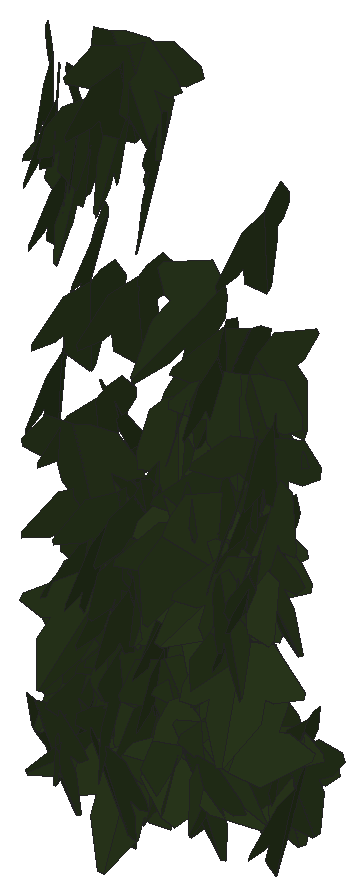
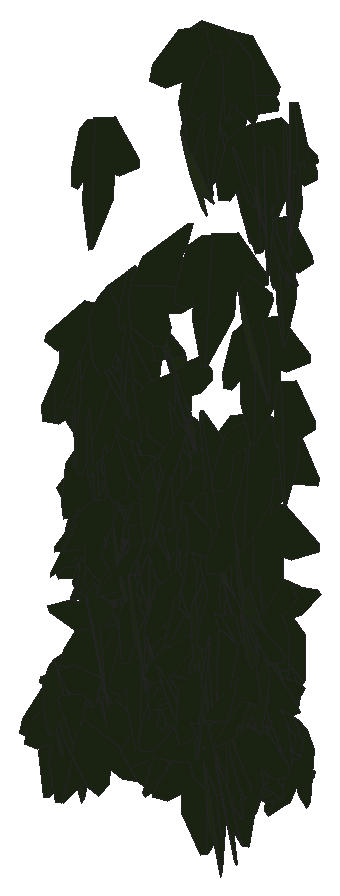
# SketchUp Ruby script. Lengths in inches.
U = 1.inch
M = Sketchup.active_model
def pt(a) = Geom::Point3d.new(a.map { |v| v * U })
def face(e, loops, mat)
  f = e.add_face(loops[0].map { |a| pt(a) })
  loops[1..].each { |l| e.add_face(l.map { |a| pt(a) }).erase! }
  f.material = f.back_material = mat if mat
  f
end
# faces: each face lists its corners as indices into pts; further lists are holes
def faces(e, pts, list, mat = nil) = list.each { |f| face(e, (f[0].is_a?(Array) ? f : [f]).map { |l| l.map { |i| pts[i] } }, mat) }
# xy, xz, yz: faces in a plane at the given z, y or x. An outline is a flat list of corners, or four numbers for a rectangle; further outlines are holes
def ring(l) = l.size == 4 ? [[l[0], l[1]], [l[2], l[1]], [l[2], l[3]], [l[0], l[3]]] : l.each_slice(2).to_a
def flat(e, list, mat, &to3) = list.each { |f| face(e, (f[0].is_a?(Array) ? f : [f]).map { |l| ring(l).map { |u, v| to3.(u, v) } }, mat) }
def xy(e, z, list, mat = nil) = flat(e, list, mat) { |x, y| [x, y, z] }
def xz(e, y, list, mat = nil) = flat(e, list, mat) { |x, z| [x, y, z] }
def yz(e, x, list, mat = nil) = flat(e, list, mat) { |y, z| [x, y, z] }
def lines(e, pts, list) = list.each { |a, b| e.add_line(pt(pts[a]), pt(pts[b])) }
# prism: a flat outline (further loops are holes) pulled along v
def prism(e, loops, v, mat = nil)
  f = face(e, loops, mat); d = Geom::Vector3d.new(v.map { |x| x * U })
  f.pushpull(f.normal.samedirection?(d) ? d.length : -d.length)
end
def box(e, o, s, mat = nil) = prism(e, [[o, [o[0] + s[0], o[1], o[2]], [o[0] + s[0], o[1] + s[1], o[2]], [o[0], o[1] + s[1], o[2]]]], [0, 0, s[2]], mat)
def at(x, y, z, deg = 0) = Geom::Transformation.translation(pt([x, y, z])) * Geom::Transformation.rotation(ORIGIN, Z_AXIS, deg.degrees)
def axes(o, x, y, z) = Geom::Transformation.new([*x, 0, *y, 0, *z, 0, *pt(o).to_a, 1])
def part(name) = M.definitions.add(name)
# library, detail: a bought-in or finely detailed component or shape, given as its bounding box
def library(name, o, s) = part(name).tap { |d| box(d.entities, o, s) }
def detail(e, o, s) = box(e.add_group.entities, o, s)
def put(e, d, t, mat = nil) = e.add_instance(d, t).tap { |i| i.material = mat if mat }
def group(e, t, mat = nil) = e.add_group.tap { |g| g.transformation = t; g.material = mat if mat }.entities
root = M.entities
M.materials.add("efeu2").color = [43, 57, 29]
c1 = part("ivyleaf_10")
p = [[0,0.5,-0.03],[-0.0625,2.02,-0.43],[-0.19,2.01,-0.46],[-0.54,1.05,-0.29],[-0.52,0.625,-0.18],[-0.83,0.76,-0.28],
  [-1.16,0.64,-0.33],[-1.15,0.33,-0.24],[-0.77,-0.39,0.02],[-0.3,-0.51,0.16],[0.04,-0.48,0.23],[-0.02,2.01,-0.4375],
  [-0.06,2.01,-0.43],[0.04,-0.49,0.23],[0.67,-0.49,0.14],[1.38,0.36,-0.2],[1.375,0.51,-0.24],[0.81,0.65,-0.19],
  [0.62,0.59,-0.15],[0.6,1.09,-0.28],[0.5,1.23,-0.31]]
faces(c1.entities,p,[[0,1,2,3,4,5,6,7,8,9,10],[11,12,0,13,14,15,16,17,18,19,20]],"efeu2")
put(root,c1,axes([515.31,136.94,182.59],[0.33871,-0.54812,-0.3443],[-0.05591,0.36236,-0.63188],[0.64487,0.31931,0.12606]))
put(root,c1,axes([515.36,137.18,180.82],[0.18828,-0.62964,-0.25162],[-0.048,0.24811,-0.65677],[0.67636,0.19288,0.02343]))
put(root,c1,axes([515.2,137.09,172.68],[-0.54988,0.28475,-0.17468],[0.14668,-0.09646,-0.61899],[-0.30013,-0.56884,0.01753]))
put(root,c1,axes([515.38,137.06,178.12],[0.1741,-0.59957,-0.27894],[-0.04764,0.27633,-0.62369],[0.65957,0.17823,0.02858]))
put(root,c1,axes([515.23,137.99,174.27],[-0.51868,0.3402,-0.19325],[0.15254,-0.11968,-0.6201],[-0.3603,-0.54042,0.01567]))
put(root,c1,axes([515.52,137.77,173.53],[0.349,0.37677,-0.38742],[-0.30336,-0.24507,-0.51163],[-0.44724,0.46025,0.04472]))
put(root,c1,axes([515.37,137.59,173.74],[0.19264,0.60685,0.10715],[-0.1052,0.143,-0.62076],[-0.6072,0.16775,0.14154]))
put(root,c1,axes([515.47,137.55,173.92],[0.58092,-0.27653,-0.19393],[-0.16516,0.10397,-0.643],[0.29462,0.60354,0.02192]))
put(root,c1,axes([515.51,136.77,182.11],[0.22554,-0.59634,-0.35365],[-0.08086,0.34673,-0.63624],[0.68859,0.23604,0.04113]))
put(root,c1,axes([515.46,137.56,175.03],[0.13649,-0.64431,0.12548],[0.01418,-0.12524,-0.6585],[0.65626,0.13671,-0.01187]))
put(root,c1,axes([515.33,137.76,173.71],[-0.01707,0.63833,-0.12351],[0.01068,-0.12326,-0.63852],[-0.65008,-0.01879,-0.00725]))
put(root,c1,axes([515.5625,137.21,181.9],[0.35337,-0.44125,-0.43697],[-0.13703,0.43497,-0.55004],[0.60569,0.35584,0.13049]))
put(root,c1,axes([515.51,137.68,173.05],[0.08292,-0.59778,0.32093],[0.07529,-0.31322,-0.60286],[0.6743,0.10849,0.02785]))
put(root,c1,axes([515.46,138.07,173.1],[0.64257,0.11943,0.00816],[-0.00384,0.0651,-0.65037],[-0.11964,0.63932,0.0647]))
put(root,c1,axes([515.57,137.65,179.83],[0.32215,-0.60836,0.03694],[0.03103,-0.02536,-0.68821],[0.60869,0.32327,0.01554]))
put(root,c1,axes([515.53,138.28,172.5],[0.42789,-0.48623,0.05749],[0.08214,-0.00397,-0.64502],[0.48268,0.43172,0.05881]))
put(root,c1,axes([515.49,137.3125,181.13],[0.55305,-0.41382,0.16129],[0.12199,-0.10614,-0.69064],[0.42706,0.56623,-0.01158]))
put(root,c1,axes([515.68,137.93,174.3],[-0.62471,0.18782,0.04065],[-0.03909,0.0112,-0.65233],[-0.18815,-0.62593,0.00053]))
put(root,c1,axes([515.69,137.32,179.13],[-0.09387,-0.66963,-0.14527],[0.02357,0.14338,-0.67617],[0.6848,-0.09673,0.00336]))
put(root,c1,axes([515.74,137.77,174.64],[0.59877,-0.12566,-0.22355],[-0.22194,0.03057,-0.61164],[0.12849,0.63841,-0.01471]))
put(root,c1,axes([515.85,137.69,173.08],[-0.57795,-0.24468,0.20168],[-0.16829,-0.11866,-0.62624],[0.26874,-0.60052,0.04156]))
put(root,c1,axes([515.96,137.73,172.47],[0.05075,0.24534,-0.60965],[-0.49643,-0.38635,-0.1968],[-0.43061,0.47432,0.15504]))
put(root,c1,axes([515.74,137.32,176.09],[-0.32489,-0.60884,-0.06624],[0.02845,0.05989,-0.69009],[0.61177,-0.32612,-0.00308]))
put(root,c1,axes([515.84,137.22,174.62],[-0.28005,-0.48958,0.37395],[-0.084,-0.37659,-0.55595],[0.6103,-0.27649,0.09508]))
put(root,c1,axes([515.79,137.34,177.41],[-0.13119,-0.65979,-0.19016],[0.02665,0.18856,-0.67263],[0.68613,-0.13348,-0.01023]))
put(root,c1,axes([515.76,137.78,175.13],[0.48977,-0.45924,-0.02017],[-0.00862,0.02029,-0.67134],[0.4596,0.48977,0.0089]))
put(root,c1,axes([515.79,138.23,172.36],[0.2756,-0.58774,-0.07754],[0.01238,0.0912,-0.64726],[0.59271,0.27138,0.04957]))
put(root,c1,axes([515.77,138.22,173.11],[0.54445,0.33969,-0.08162],[-0.08031,-0.02539,-0.64139],[-0.34,0.54995,0.0208]))
put(root,c1,axes([515.92,137.05,182.08],[-0.16433,-0.70047,-0.06187],[0.01857,0.05919,-0.71947],[0.70295,-0.16531,0.00455]))
put(root,c1,axes([515.96,136.84,177.25],[-0.68545,-0.12976,-0.01894],[0.0189,0.00199,-0.69762],[0.12976,-0.68571,0.00156]))
put(root,c1,axes([515.99,138.04,173.74],[-0.14545,-0.63951,0.10688],[0.0004,-0.10962,-0.65539],[0.64838,-0.14339,0.02438]))
put(root,c1,axes([516.13,138.01,174.14],[-0.40383,0.39671,0.35406],[-0.29855,0.19874,-0.5632],[-0.44001,-0.49894,0.05718]))
put(root,c1,axes([516.05,138.08,172.52],[-0.57007,-0.29009,0.06256],[-0.04937,-0.0409,-0.63948],[0.29262,-0.57204,0.01399]))
put(root,c1,axes([516.02,137.14,175.65],[0.23214,-0.67517,-0.16839],[-0.0297,0.16773,-0.7135],[0.69522,0.23261,0.02574]))
put(root,c1,axes([516.09,137.77,173.36],[-0.63952,-0.08182,0.08241],[-0.07285,-0.07655,-0.64133],[0.09043,-0.64025,0.06615]))
put(root,c1,axes([516.07,137.54,174.79],[-0.01294,-0.62664,-0.24537],[0.03214,0.24456,-0.62627],[0.6722,-0.02376,0.02522]))
put(root,c1,axes([516.14,138.02,174.81],[0.2194,-0.62079,-0.10657],[0.00444,0.11437,-0.6571],[0.62986,0.21544,0.04176]))
put(root,c1,axes([516.25,137.29,176.19],[-0.34841,-0.57057,-0.12086],[0.05321,0.1091,-0.66844],[0.5808,-0.35227,-0.01126]))
put(root,c1,axes([516.38,137.875,173.91],[-0.38278,-0.5273,0.0378],[-0.02134,-0.03121,-0.65159],[0.52822,-0.38337,0.00106]))
put(root,c1,axes([516.26,137.2,182],[0.52787,-0.47279,-0.01699],[0.0045,0.03047,-0.70818],[0.47307,0.52726,0.02569]))
put(root,c1,axes([516.09,137.51,173.46],[0.23481,-0.45598,0.45044],[0.28413,-0.35595,-0.50845],[0.57453,0.36239,0.06735]))
put(root,c1,axes([515.97,137.84,176.6875],[-0.42605,0.12559,0.55668],[0.5071,-0.23535,0.44119],[0.26177,0.66032,0.05137]))
put(root,c1,axes([516.33,136.99,172.51],[-0.57322,0.29702,-0.00692],[0.00683,-0.00187,-0.6456],[-0.29702,-0.57326,-0.00148]))
put(root,c1,axes([516.75,137.3125,176.05],[-0.44733,0.03746,-0.51049],[-0.50777,0.05308,0.44884],[0.06459,0.67667,-0.00695]))
put(root,c1,axes([516.29,137.35,172.19],[0.71633,-0.04816,-0.04057],[-0.03949,0.01731,-0.7178],[0.04905,0.71727,0.0146]))
put(root,c1,axes([516.44,138.03,173.33],[-0.3324,-0.57437,0.05078],[0.02629,-0.07365,-0.66095],[0.57602,-0.32809,0.05947]))
put(root,c1,axes([516.31,137.68,172.94],[0.07524,0.3696,0.54415],[0.01485,0.54661,-0.37332],[-0.65764,0.05463,0.05383]))
put(root,c1,axes([516.47,137.21,174.89],[0.05804,-0.57536,-0.35999],[0.03521,0.36337,-0.57509],[0.67779,0.03039,0.0607]))
put(root,c1,axes([516.43,137.33,175.47],[-0.20436,-0.50261,-0.45725],[0.16344,0.4271,-0.54251],[0.65953,-0.26157,-0.00724]))
put(root,c1,axes([517,137.38,174.7],[0.09853,0.07319,-0.70142],[-0.70214,0.0764,-0.09066],[0.06593,0.70418,0.08274]))
put(root,c1,axes([516.51,137.99,175.35],[0.09012,0.55236,-0.35938],[-0.12441,-0.34194,-0.55675],[-0.64713,0.14266,0.05699]))
put(root,c1,axes([516.6,136.85,182.93],[-0.10855,-0.66403,-0.28612],[0.0283,0.2852,-0.67263],[0.72249,-0.11094,-0.01664]))
put(root,c1,axes([516.43,137.83,173.96],[-0.21607,-0.49266,-0.36988],[0.24805,0.28922,-0.53013],[0.56391,-0.31599,0.09146]))
put(root,c1,axes([516.6,137.25,176.36],[-0.12219,-0.5641,-0.39116],[0.09299,0.38004,-0.57712],[0.68012,-0.15331,0.00863]))
put(root,c1,axes([516.63,137.64,173.25],[-0.06443,-0.59383,-0.28635],[0.07386,0.2794,-0.59604],[0.65512,-0.0899,0.03904]))
put(root,c1,axes([516.59,138.08,173.53],[0.6626,-0.01612,-0.00916],[-0.0091,0.00268,-0.66279],[0.01616,0.66265,0.00246]))
put(root,c1,axes([516.875,137.71,177.12],[-0.27266,0.39824,0.45446],[-0.26,0.37274,-0.48263],[-0.54546,-0.37675,0.00288]))
put(root,c1,axes([516.64,136.91,183.27],[-0.674,0.13808,-0.21923],[0.19219,-0.1433,-0.68112],[-0.17375,-0.69412,0.097]))
put(root,c1,axes([516.87,137.97,176.09],[0.61823,0.04994,-0.24838],[-0.25131,0.20381,-0.58455],[0.03208,0.63432,0.20737]))
put(root,c1,axes([516.83,136.875,183.25],[-0.60221,-0.37852,-0.095],[0.0687,0.06915,-0.71095],[0.38416,-0.60572,-0.02179]))
put(root,c1,axes([516.89,136.82,179.84],[-0.11494,-0.69555,-0.19295],[0.03206,0.19027,-0.70498],[0.72111,-0.11932,0.00059]))
put(root,c1,axes([516.71,138.24,173.8125],[0.50861,-0.37359,0.17246],[0.1402,-0.10045,-0.63107],[0.38686,0.52758,0.00197]))
put(root,c1,axes([517.09,137.91,172.15],[0.11225,0.27553,0.57456],[-0.23243,-0.52551,0.29741],[0.59331,-0.258,0.00781]))
put(root,c1,axes([516.98,137.92,176.64],[0.07944,-0.65598,0.04507],[0.00925,-0.04428,-0.66076],[0.65746,0.07988,0.00385]))
put(root,c1,axes([517.03,137.17,174.21],[0.19579,-0.55272,-0.3456],[-0.03576,0.3512,-0.58194],[0.65089,0.18556,0.07198]))
put(root,c1,axes([517.0625,137.38,174.79],[0.13093,-0.64723,-0.20686],[-0.04903,0.20112,-0.66029],[0.67771,0.13959,-0.00781]))
put(root,c1,axes([517,137.93,175.19],[-0.5254,-0.35416,-0.188],[0.14126,0.12652,-0.63313],[0.37526,-0.54349,-0.02488]))
put(root,c1,axes([517.12,137.18,172.875],[0.44878,-0.44902,-0.14413],[-0.09723,0.10658,-0.63481],[0.46146,0.45915,0.00641]))
put(root,c1,axes([517.15,137.9,176.62],[-0.60853,0.26913,0.0819],[-0.06744,0.04992,-0.66513],[-0.27311,-0.61198,-0.01824]))
put(root,c1,axes([516.9,137.28,181.91],[0.35879,-0.49456,0.39986],[0.2629,-0.3027,-0.61029],[0.5791,0.44384,0.02932]))
put(root,c1,axes([517.18,137.47,175.08],[-0.02902,-0.59884,-0.35837],[0.03346,0.35707,-0.59938],[0.69708,-0.04207,0.01385]))
put(root,c1,axes([517.23,137.96,173.86],[-0.10834,-0.62211,-0.16859],[0.01456,0.16855,-0.63131],[0.64438,-0.10841,-0.01408]))
put(root,c1,axes([517.29,137.3,176.04],[-0.26212,-0.59598,0.10222],[0.01025,-0.11577,-0.64872],[0.6046,-0.25642,0.05531]))
put(root,c1,axes([517.3125,138.02,174.8125],[0.26285,-0.58889,-0.16814],[-0.04203,0.1652,-0.64428],[0.61098,0.26471,0.02802]))
put(root,c1,axes([517.32,137.41,175.66],[-0.63696,0.21757,0.00256],[-0.00241,0.00085,-0.6731],[-0.21757,-0.63697,-0.00003]))
put(root,c1,axes([517.33,137.15,178.11],[0.43383,-0.53894,-0.01151],[-0.00982,0.00686,-0.69185],[0.53898,0.43392,-0.00335]))
put(root,c1,axes([517.26,137.86,175.47],[0.00628,0.67482,-0.04731],[-0.00604,-0.04725,-0.67483],[-0.67645,0.00669,0.00558]))
put(root,c1,axes([517.3125,137.1,174.09],[-0.58587,-0.2297,-0.17629],[0.18628,0.00562,-0.62638],[0.22168,-0.6118,0.06044]))
put(root,c1,axes([517.32,137.21,177.85],[0.18438,0.64508,-0.10771],[-0.01917,-0.10653,-0.67083],[-0.65373,0.18506,-0.01071]))
put(root,c1,axes([517.06,137.375,176.97],[-0.13667,0.10033,-0.66092],[0.41354,-0.51733,-0.16405],[-0.52522,-0.43343,0.04281]))
put(root,c1,axes([517.43,137.54,179.54],[-0.04678,-0.25073,0.67973],[0.11574,-0.67498,-0.24101],[0.71519,0.09283,0.08347]))
put(root,c1,axes([517.57,137.73,173.8125],[-0.18975,-0.57246,0.28821],[-0.00179,-0.3001,-0.59726],[0.64091,-0.17032,0.08366]))
put(root,c1,axes([517.54,137.33,176.41],[0.59834,0.24749,-0.13382],[-0.11974,-0.06059,-0.64743],[-0.2546,0.61012,-0.01001]))
put(root,c1,axes([517.61,137.73,175.67],[0.64542,0.09393,-0.12404],[-0.13078,0.04074,-0.64963],[-0.0843,0.65597,0.05811]))
put(root,c1,axes([517.73,137.51,176.92],[-0.15315,-0.62134,0.23451],[-0.04825,-0.22961,-0.63989],[0.66237,-0.1604,0.00761]))
put(root,c1,axes([517.78,138.24,172.49],[-0.08365,-0.45227,0.45421],[-0.10619,-0.44196,-0.45962],[0.63212,-0.13409,-0.0171]))
put(root,c1,axes([517.54,137.9,175.28],[0.48232,-0.46295,0.05336],[0.12111,0.05037,-0.65772],[0.45001,0.48264,0.11982]))
put(root,c1,axes([517.7,137.84,175.3],[0.28475,-0.59519,-0.0542],[-0.0181,0.05142,-0.65978],[0.59738,0.28527,0.00584]))
put(root,c1,axes([517.73,137.05,172.83],[-0.62943,0.18675,-0.06649],[0.06124,-0.02732,-0.65649],[-0.18854,-0.63234,0.00873]))
put(root,c1,axes([517.46,136.93,173.23],[-0.08017,-0.27202,-0.62845],[0.4499,0.45611,-0.25481],[0.51627,-0.43971,0.12447]))
put(root,c1,axes([518.28,138,173.26],[0.08216,0.10062,-0.64304],[-0.64415,-0.08031,-0.09487],[-0.09327,0.64328,0.08874]))
put(root,c1,axes([517.98,137.57,179.02],[-0.07792,-0.68304,0.24413],[-0.01124,-0.24437,-0.6873],[0.72527,-0.07717,0.01558]))
put(root,c1,axes([517.88,137.6,173.18],[-0.02995,-0.53898,0.41742],[0.11967,-0.41549,-0.5279],[0.67113,0.05004,0.11276]))
put(root,c1,axes([518.03,137.08,179.01],[0.09263,-0.58298,-0.4239],[-0.03229,0.4236,-0.58962],[0.72008,0.09399,0.02809]))
put(root,c1,axes([517.9,137.86,175.87],[0.16478,0.65327,-0.02323],[-0.06767,-0.00678,-0.67069],[-0.65017,0.16627,0.06392]))
put(root,c1,axes([517.82,136.53,176.49],[-0.11089,-0.54035,-0.57495],[0.32929,0.49593,-0.52959],[0.71702,-0.31132,0.1543]))
put(root,c1,axes([517.57,136.89,173.02],[0.32001,0.18948,0.5792],[0.46056,0.35322,-0.37001],[-0.39908,0.55957,0.03743]))
put(root,c1,axes([518.25,137.17,175.88],[0.48106,0.23471,-0.44909],[-0.43071,-0.13683,-0.53288],[-0.26695,0.64372,0.05048]))
put(root,c1,axes([517.97,137.2,175.49],[0.65876,0.21686,-0.05702],[-0.05384,-0.01879,-0.69354],[-0.21767,0.66096,-0.00101]))
put(root,c1,axes([518.07,137.82,177.79],[-0.66777,0.09926,-0.07014],[0.06718,-0.025,-0.67495],[-0.10129,-0.67098,0.01477]))
put(root,c1,axes([518.06,138.04,174.17],[0.34254,-0.57038,-0.01055],[0.0322,0.03162,-0.66388],[0.56957,0.34124,0.04388]))
put(root,c1,axes([517.99,137.66,177.05],[0.56864,-0.37135,0.07596],[0.11013,0.03082,-0.67376],[0.36268,0.57287,0.08549]))
put(root,c1,axes([518.27,136.95,176.82],[0.35463,-0.5377,-0.25259],[-0.13853,0.21122,-0.64412],[0.5777,0.38073,0.0006]))
put(root,c1,axes([518.22,137.38,178.51],[-0.59204,-0.36167,0.04779],[0.03562,-0.14797,-0.67855],[0.36307,-0.57524,0.1445]))
put(root,c1,axes([518.11,137.61,177.82],[0.51476,-0.43525,0.05594],[0.06637,-0.00802,-0.67311],[0.43378,0.51772,0.0366]))
put(root,c1,axes([517.97,138.02,173.01],[0.60323,0.21911,0.16144],[0.15375,0.04958,-0.64176],[-0.22458,0.62249,-0.00572]))
put(root,c1,axes([518.27,137.32,175.81],[-0.23743,-0.60996,0.18085],[0.01854,-0.19958,-0.64881],[0.63593,-0.22192,0.08644]))
put(root,c1,axes([518.18,138.2,172.59],[-0.46617,-0.43377,-0.11788],[0.14543,0.01515,-0.63087],[0.42533,-0.48061,0.08651]))
put(root,c1,axes([518.16,137.99,175.72],[0.02349,0.60291,-0.28232],[-0.00929,-0.28217,-0.60336],[-0.66567,0.02521,-0.00154]))
put(root,c1,axes([518.34,137.24,175.48],[0.18811,-0.58742,-0.25252],[-0.04433,0.2506,-0.61599],[0.63786,0.19065,0.03165]))
put(root,c1,axes([518.35,137.78,176.4],[-0.03838,-0.67635,-0.02533],[0.00013,0.02536,-0.67743],[0.67682,-0.03836,-0.0013]))
put(root,c1,axes([518.31,137.66,177.02],[0.20102,-0.63737,-0.12925],[0.01867,0.14088,-0.6657],[0.65007,0.19305,0.05908]))
put(root,c1,axes([518.15,137.81,175.82],[-0.55173,0.22528,-0.30258],[0.27147,-0.13514,-0.59561],[-0.26194,-0.61457,0.02005]))
put(root,c1,axes([518.36,137.78,178.69],[-0.04238,0.56585,0.36736],[-0.1292,0.35447,-0.56089],[-0.66216,-0.10538,0.08593]))
put(root,c1,axes([518.47,137.51,177.63],[-0.51872,-0.43226,0.04725],[-0.03394,-0.03307,-0.67521],[0.43351,-0.51981,0.00367]))
put(root,c1,axes([518.43,137.32,175.75],[0.00556,-0.60267,-0.36624],[0.07553,0.36465,-0.59891],[0.70117,-0.0345,0.06741]))
put(root,c1,axes([518.48,138.24,173.08],[0.08316,-0.64572,0.0393],[-0.00287,-0.03999,-0.65101],[0.64691,0.08283,-0.00794]))
put(root,c1,axes([518.46,138.09,172.64],[-0.31211,-0.53525,-0.20674],[0.0996,0.18123,-0.61958],[0.56508,-0.32757,-0.00498]))
put(root,c1,axes([518.37,136.8,175.16],[-0.10914,-0.47043,-0.50662],[0.25275,0.45023,-0.47252],[0.64349,-0.25663,0.09967]))
put(root,c1,axes([518.42,136.84,175.74],[-0.17014,0.63679,-0.08319],[0.01668,-0.08165,-0.65911],[-0.64199,-0.17088,0.00493]))
put(root,c1,axes([518.46,137.6,176.89],[0.63603,-0.21604,-0.00368],[-0.00339,0.00146,-0.67172],[0.21604,0.63604,0.0003]))
put(root,c1,axes([518.51,136.95,174.71],[0.40459,0.5108,-0.1252],[-0.07946,-0.09677,-0.65162],[-0.51988,0.41232,0.00216]))
put(root,c1,axes([518.56,137.57,177.85],[0.20283,-0.61472,-0.22205],[0.0762,0.25315,-0.63122],[0.64914,0.16236,0.14348]))
put(root,c1,axes([518.67,137.23,181.29],[0.04153,-0.67012,-0.24624],[0.00122,0.24672,-0.67122],[0.71392,0.03856,0.01547]))
put(root,c1,axes([518.6875,137.76,172.37],[0.13106,-0.62894,-0.11532],[-0.03508,0.11047,-0.64235],[0.63846,0.13517,-0.01162]))
put(root,c1,axes([518.41,137.1,173.45],[0.72153,0.03371,-0.16606],[0.16469,0.03136,0.72195],[0.03986,-0.73973,0.02304]))
